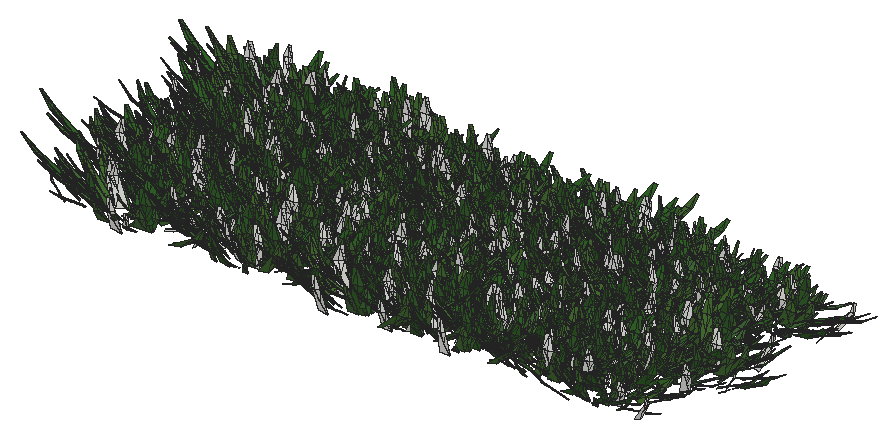
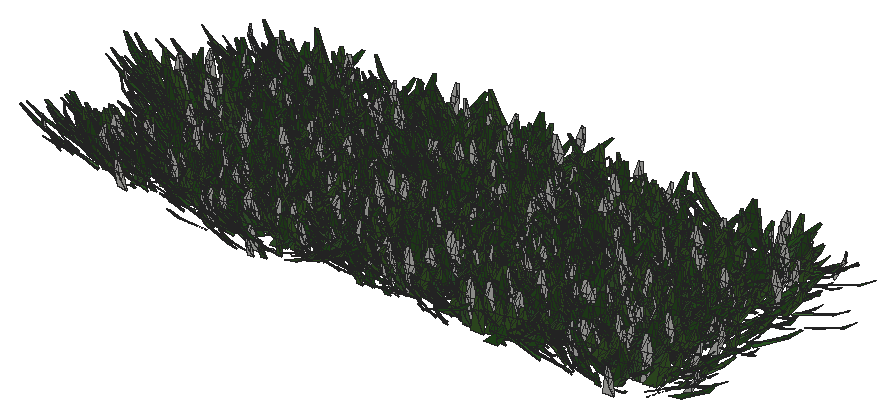
# SketchUp Ruby script. Lengths in inches.
U = 1.inch
M = Sketchup.active_model
def pt(a) = Geom::Point3d.new(a.map { |v| v * U })
def face(e, loops, mat)
  f = e.add_face(loops[0].map { |a| pt(a) })
  loops[1..].each { |l| e.add_face(l.map { |a| pt(a) }).erase! }
  f.material = f.back_material = mat if mat
  f
end
# faces: each face lists its corners as indices into pts; further lists are holes
def faces(e, pts, list, mat = nil) = list.each { |f| face(e, (f[0].is_a?(Array) ? f : [f]).map { |l| l.map { |i| pts[i] } }, mat) }
# xy, xz, yz: faces in a plane at the given z, y or x. An outline is a flat list of corners, or four numbers for a rectangle; further outlines are holes
def ring(l) = l.size == 4 ? [[l[0], l[1]], [l[2], l[1]], [l[2], l[3]], [l[0], l[3]]] : l.each_slice(2).to_a
def flat(e, list, mat, &to3) = list.each { |f| face(e, (f[0].is_a?(Array) ? f : [f]).map { |l| ring(l).map { |u, v| to3.(u, v) } }, mat) }
def xy(e, z, list, mat = nil) = flat(e, list, mat) { |x, y| [x, y, z] }
def xz(e, y, list, mat = nil) = flat(e, list, mat) { |x, z| [x, y, z] }
def yz(e, x, list, mat = nil) = flat(e, list, mat) { |y, z| [x, y, z] }
def lines(e, pts, list) = list.each { |a, b| e.add_line(pt(pts[a]), pt(pts[b])) }
# prism: a flat outline (further loops are holes) pulled along v
def prism(e, loops, v, mat = nil)
  f = face(e, loops, mat); d = Geom::Vector3d.new(v.map { |x| x * U })
  f.pushpull(f.normal.samedirection?(d) ? d.length : -d.length)
end
def box(e, o, s, mat = nil) = prism(e, [[o, [o[0] + s[0], o[1], o[2]], [o[0] + s[0], o[1] + s[1], o[2]], [o[0], o[1] + s[1], o[2]]]], [0, 0, s[2]], mat)
def at(x, y, z, deg = 0) = Geom::Transformation.translation(pt([x, y, z])) * Geom::Transformation.rotation(ORIGIN, Z_AXIS, deg.degrees)
def axes(o, x, y, z) = Geom::Transformation.new([*x, 0, *y, 0, *z, 0, *pt(o).to_a, 1])
def part(name) = M.definitions.add(name)
# library, detail: a bought-in or finely detailed component or shape, given as its bounding box
def library(name, o, s) = part(name).tap { |d| box(d.entities, o, s) }
def detail(e, o, s) = box(e.add_group.entities, o, s)
def put(e, d, t, mat = nil) = e.add_instance(d, t).tap { |i| i.material = mat if mat }
def group(e, t, mat = nil) = e.add_group.tap { |g| g.transformation = t; g.material = mat if mat }.entities
root = M.entities
M.materials.add("Material82").color = [68, 110, 58]
M.materials.add("Material83").color = [48, 90, 38]
M.materials.add("Material84").color = [68, 110, 48]
M.materials.add("Material85").color = [48, 90, 48]
M.materials.add("Material86").color = [58, 110, 58]
M.materials.add("Material87").color = [58, 90, 38]
M.materials.add("Material88").color = [68, 100, 58]
M.materials.add("Material89").color = [48, 100, 38]
c1 = part("grass00")
p = [[-0.6875,0.15,0],[-0.56,0.08,5.52],[-0.04,0.03,2.76],[0.48,-0.02,0],[0.35,-0.02,5.52],[-0.1,-0.14,5.52],
  [-0.12,0.65,8.37],[-0.42,0.65,8.37]]
faces(c1.entities,p,[[0,1,2,3],[3,2,4],[1,5,2],[5,4,2],[1,6,5],[4,5,6],[7,6,1]])
c2 = part("Group16\#1")
put(c2.entities,c1,axes([1.44,-0.61,-0.01],[0.05352,0.12609,0],[-0.10704,0.04543,0.07239],[0.06664,-0.02828,0.11628]),"Material85")
put(c2.entities,c1,axes([0.76,-0.15,-0.01],[0.04676,0.24062,0],[-0.23162,0.04501,0.06642],[0.0652,-0.01267,0.23595]),"Material82")
put(c2.entities,c1,axes([0.79,0.01,-0.01],[-0.00606,0.34651,0],[-0.34381,-0.00602,0.0432],[0.04319,0.00076,0.34386]))
put(c2.entities,c1,axes([1,0.23,-0.01],[-0.07192,0.31144,0],[-0.28722,-0.06632,0.1236],[0.12043,0.02781,0.29478]),"Material84")
put(c2.entities,c1,axes([1.66,0.77,-0.01],[-0.13828,0.29651,0],[-0.21551,-0.1005,0.22471],[0.20365,0.09498,0.23779]),"Material89")
put(c2.entities,c1,axes([0.6875,0.52,-0.01],[-0.18126,0.24051,0],[-0.22746,-0.17142,0.09788],[0.07817,0.05891,0.28481]),"Material84")
put(c2.entities,c1,axes([0.68,0.78,-0.01],[-0.215,0.18688,0],[-0.12385,-0.14248,0.21334],[0.13995,0.16101,0.18878]),"Material82")
put(c2.entities,c1,axes([0.56,1,-0.01],[-0.13756,0.07624,0],[-0.06159,-0.11112,0.0927],[0.04494,0.08108,0.12705]),"Material84")
put(c2.entities,c1,axes([0.2,0.64,-0.01],[-0.23729,0.07254,0],[-0.05711,-0.18681,0.153],[0.04473,0.14632,0.19535]),"Material89")
put(c2.entities,c1,axes([0.0625,0.72,-0.01],[-0.28874,0.02525,0],[-0.02179,-0.24916,0.14647],[0.01276,0.14591,0.25012]),"Material82")
put(c2.entities,c1,axes([-0.08,0.62,-0.01],[-0.34089,-0.04187,0],[0.03255,-0.26504,0.216],[-0.02633,0.21439,0.26703]),"Material89")
put(c2.entities,c1,axes([-0.34,0.98,-0.01],[-0.14314,-0.0493,0],[0.04397,-0.12769,0.06843],[-0.02228,0.0647,0.13505]),"Material89")
put(c2.entities,c1,axes([-0.87,1.45,-0.01],[-0.23488,-0.14114,0],[0.13761,-0.22901,0.06087],[-0.03135,0.05217,0.26717]))
put(c2.entities,c1,axes([-0.72,0.77,-0.01],[-0.14208,-0.13251,0],[0.07209,-0.0773,0.16301],[-0.11118,0.11922,0.1057]),"Material89")
put(c2.entities,c1,axes([-0.62,0.43,-0.01],[-0.14845,-0.21203,0],[0.18654,-0.13061,0.12304],[-0.10079,0.07057,0.22772]),"Material82")
put(c2.entities,c1,axes([-0.68,0.29,-0.01],[-0.13639,-0.32136,0],[0.31723,-0.13464,0.05579],[-0.05136,0.0218,0.34462]),"Material83")
put(c2.entities,c1,axes([-0.64,0.125,-0.01],[-0.0458,-0.23569,0],[0.22124,-0.043,0.08276],[-0.08124,0.01579,0.22538]),"Material86")
put(c2.entities,c1,axes([-1.6,-0.03,-0.01],[0.00576,-0.32897,0],[0.27526,0.00482,0.18018],[-0.18015,-0.00315,0.2753]),"Material84")
put(c2.entities,c1,axes([-1.36,-0.31,-0.01],[0.05718,-0.24765,0],[0.18172,0.04196,0.17267],[-0.16825,-0.03885,0.1865]),"Material89")
put(c2.entities,c1,axes([-1.54,-0.72,-0.01],[0.06537,-0.14017,0],[0.13555,0.06321,0.03939],[-0.0357,-0.01665,0.14956]))
put(c2.entities,c1,axes([-1.19,-0.9,-0.01],[0.09597,-0.12735,0],[0.11214,0.08451,0.07557],[-0.06035,-0.04548,0.14042]),"Material88")
put(c2.entities,c1,axes([-0.47,-0.54,-0.01],[0.11588,-0.10072,0],[0.0618,0.0711,0.12124],[-0.07953,-0.0915,0.0942]))
put(c2.entities,c1,axes([-0.47,-0.84,-0.01],[0.11927,-0.0661,0],[0.06603,0.11913,0.00646],[-0.00313,-0.00565,0.13621]),"Material84")
put(c2.entities,c1,axes([-0.38,-1.24,-0.01],[0.28037,-0.08571,0],[0.0618,0.20215,0.20315],[-0.05939,-0.19428,0.21139]),"Material88")
put(c2.entities,c1,axes([-0.06,-0.66,-0.01],[0.22719,-0.01987,0],[0.01247,0.14255,0.17758],[-0.01547,-0.17691,0.1431]),"Material87")
put(c2.entities,c1,axes([0.11,-0.89,-0.01],[0.14882,0.01828,0],[-0.01058,0.08611,0.12229],[0.01491,-0.12138,0.08676]),"Material85")
put(c2.entities,c1,axes([0.25,-0.72,-0.01],[0.20481,0.07053,0],[-0.06206,0.18022,0.10291],[0.03351,-0.0973,0.1906]),"Material85")
put(c2.entities,c1,axes([0.85,-1.42,-0.01],[0.16481,0.09904,0],[-0.09472,0.15762,0.05616],[0.02893,-0.04814,0.18389]),"Material84")
put(c2.entities,c1,axes([1.01,-1.09,-0.01],[0.21858,0.20385,0],[-0.17495,0.1876,0.15339],[0.10462,-0.11218,0.25652]),"Material89")
put(c2.entities,c1,axes([1.01,-0.71,-0.01],[0.08733,0.12473,0],[-0.06445,0.04512,0.13037],[0.1068,-0.07477,0.07867]),"Material85")
c3 = part("Group15\#1")
put(c3.entities,c2,at(0,0,0))
c4 = part("3darcstudiotree_grass00\#1")
put(c4.entities,c3,at(0,0,0))
put(root,c4,axes([1754.14,355.86,-34.17],[-3.58056,-0.39826,0],[0.95821,-1.33984,-0.015],[0.02011,-0.02812,1.30652]))
put(root,c4,axes([1754,346.47,-34.17],[-3.11874,1.35551,0],[-2.91461,-1.04296,-0.0082],[-0.03562,-0.01275,1.73071]))
put(root,c4,axes([1755.32,353.64,-34.17],[-3.23633,-0.50825,0],[1.72306,-1.70642,-0.01803],[0.03469,-0.03435,1.81493]))
put(root,c4,axes([1754.23,365.84,-34.17],[-1.77081,1.15286,0],[-3.98211,-0.9513,-0.05645],[-0.27396,-0.06545,1.97994]))
put(root,c4,axes([1754.09,364.16,-34.17],[2.97915,0.86965,0],[-2.38175,1.26898,-0.05487],[-0.15774,0.08404,1.44987]))
put(root,c4,axes([1755.32,361.99,-34.17],[3.36447,-1.00796,0],[2.1967,1.14039,-0.03309],[0.10605,0.05506,1.44206]))
put(root,c4,axes([1756.76,350.61,-34.17],[-3.57677,-1.09741,0],[2.84767,-1.44352,-0.06227],[0.15089,-0.07649,1.37168]))
put(root,c4,axes([1755.63,340.29,-34.17],[-0.9025,1.72738,0],[-3.54084,-0.28772,-0.03296],[-0.16809,-0.01366,1.411]))
put(root,c4,axes([1755.79,359.44,-34.17],[-1.59741,1.49736,0],[-3.22806,-0.5356,-0.02216],[-0.12937,-0.02146,1.66252]))
put(root,c4,axes([1756.57,348.21,-34.17],[-0.7508,1.54691,0],[-4.43091,-0.33447,-0.01652],[-0.07223,-0.00545,1.50529]))
put(root,c4,axes([1756.76,368.2,-34.17],[4.00478,-0.12141,0],[0.32544,1.66956,-0.03486],[0.01415,0.07259,1.68524]))
put(root,c4,axes([1757.17,357.11,-34.17],[3.83024,1.03121,0],[-2.22146,1.2833,-0.02215],[-0.08012,0.04629,1.8946]))
put(root,c4,axes([1760.06,353.15,-34.17],[-3.68156,-0.36216,0],[0.87025,-1.37591,-0.04204],[0.06138,-0.09705,1.62585]))
put(root,c4,axes([1759.72,339.76,-34.17],[-3.79448,1.12109,0],[-2.55555,-1.34526,-0.03017],[-0.0978,-0.05148,1.72726]))
put(root,c4,axes([1760.08,363.96,-34.17],[-3.10715,1.0196,0],[-2.89034,-1.36991,-0.01948],[-0.06651,-0.03152,1.80807]))
put(root,c4,axes([1760.29,361.45,-34.17],[3.31286,-0.55128,0],[1.80617,1.68812,-0.0407],[0.06877,0.06427,1.51351]))
put(root,c4,axes([1759.56,342.87,-34.17],[3.22227,0.82324,0],[-2.17222,1.32236,-0.01048],[-0.0296,0.01802,1.55517]))
put(root,c4,axes([1761.71,359.76,-34.17],[-4.269,-0.81813,0],[1.88917,-1.53314,-0.01545],[0.03796,-0.03081,1.8215]))
put(root,c4,axes([1760.42,355.12,-34.17],[0.15057,1.31453,0],[-3.70176,0.06595,-0.0329],[-0.23461,0.00418,1.98251]))
put(root,c4,axes([1760.38,347.21,-34.17],[-0.68682,1.71759,0],[-4.33467,-0.26958,-0.03641],[-0.15889,-0.00988,1.45326]))
put(root,c4,axes([1760.8,348.04,-34.17],[-1.33529,1.77622,0],[-3.16975,-0.37061,-0.00114],[-0.00828,-0.00097,1.86907]))
put(root,c4,axes([1760.34,356.7,-34.17],[1.34239,1.63135,0],[-4.02681,0.51535,-0.01715],[-0.07258,0.00929,1.41194]))
put(root,c4,axes([1761.43,366.09,-34.17],[-1.89402,1.2029,0],[-3.60721,-0.88336,-0.02009],[-0.09037,-0.02213,1.68525]))
put(root,c4,axes([1762.37,350.73,-34.17],[2.81192,0.87479,0],[-2.84329,1.42145,-0.06164],[-0.14998,0.07498,1.3518]))
put(root,c4,axes([1762.7,344.07,-34.17],[0.48103,1.53156,0],[-4.51259,0.22043,-0.03401],[-0.13914,0.0068,1.40523]))
put(root,c4,axes([1765.1875,360.96,-34.17],[-3.65599,0.07986,0],[-0.21877,-1.55768,-0.04105],[-0.01403,-0.0999,1.83253]))
put(root,c4,axes([1765.81,350.74,-34.17],[-2.36391,-1.30666,0],[2.88424,-0.81154,-0.04134],[0.24623,-0.06928,1.943]))
put(root,c4,axes([1765.08,345.07,-34.17],[-2.91503,0.96344,0],[-2.99535,-1.40954,-0.01682],[-0.05566,-0.02619,1.80026]))
put(root,c4,axes([1765.88,349.41,-34.17],[2.5477,-1.31265,0],[2.99582,0.90433,-0.00025],[0.00104,0.00031,1.45509]))
put(root,c4,axes([1765.71,363.8125,-34.17],[2.84002,-1.42543,0],[3.17904,0.98511,-0.04001],[0.1906,0.05906,1.83572]))
put(root,c4,axes([1765.02,357.56,-34.17],[4.10776,0.45174,0],[-0.96091,1.35899,-0.03867],[-0.06802,0.0962,1.75619]))
put(root,c4,axes([1766.99,355.55,-34.17],[-3.02492,-1.16677,0],[2.80082,-1.12934,-0.0483],[0.17838,-0.07192,1.58573]))
put(root,c4,axes([1767.42,342.88,-34.17],[1.67083,-1.60234,0],[3.7829,0.6135,-0.00107],[0.00454,0.00074,1.41133]))
put(root,c4,axes([1767.01,352.8125,-34.17],[-1.6341,1.38385,0],[-3.29524,-0.60518,-0.01596],[-0.09907,-0.01819,1.86544]))
put(root,c4,axes([1767.25,358.875,-34.17],[-1.88391,1.25543,0],[-3.77395,-0.8808,-0.04665],[-0.1806,-0.04215,1.47851]))
put(root,c4,axes([1767.61,346.4375,-34.17],[2.32026,0.93484,0],[-2.86948,1.10768,-0.01876],[-0.07886,0.03044,1.77063]))
put(root,c4,axes([1768.34,365.39,-34.17],[0.18236,1.53314,0],[-4.12116,0.07624,-0.04808],[-0.2649,0.0049,1.70557]))
put(root,c4,axes([1770.02,352.5,-34.17],[-3.65717,1.04753,0],[-2.10189,-1.14131,-0.02785],[-0.11272,-0.06121,1.84622]))
put(root,c4,axes([1770,363.99,-34.17],[2.69686,-1.18339,0],[2.47302,0.87653,-0.01288],[0.05957,0.02111,1.54961]))
put(root,c4,axes([1770.875,357.19,-34.17],[-3.84397,-0.38485,0],[1.07963,-1.67717,-0.00944],[0.01366,-0.02122,1.93444]))
put(root,c4,axes([1770.72,350.7,-34.17],[-1.0379,-1.53247,0],[3.79206,-0.39944,-0.04991],[0.21721,-0.02288,1.32514]))
put(root,c4,axes([1770.86,348.89,-34.17],[1.97874,-1.59829,0],[3.60248,0.69366,-0.03421],[0.19371,0.0373,1.89316]))
put(root,c4,axes([1770.07,366.47,-34.17],[1.07752,1.49554,0],[-4.17421,0.46775,-0.01918],[-0.10688,0.01198,1.88463]))
put(root,c4,axes([1772.22,346.51,-34.17],[-0.05891,-1.32731,0],[4.1482,-0.02863,-0.04239],[0.194,-0.00134,1.42343]))
put(root,c4,axes([1773.02,362.16,-34.17],[-0.12973,-1.5282,0],[4.23676,-0.05594,-0.02714],[0.12341,-0.00163,1.44559]))
put(root,c4,axes([1772.64,340.54,-34.17],[2.6038,-1.3441,0],[3.00735,0.90609,-0.00592],[0.02965,0.00893,1.78738]))
put(root,c4,axes([1773.5,341.58,-34.17],[-2.61082,-1.14432,0],[2.90627,-1.03127,-0.02928],[0.10098,-0.03583,1.35967]))
put(root,c4,axes([1772.72,367.58,-34.17],[-0.14307,1.431,0],[-4.32963,-0.06732,-0.01193],[-0.07261,-0.00113,1.97773]))
put(root,c4,axes([1773.49,355.81,-34.17],[-0.09674,1.30199,0],[-3.40883,-0.03939,-0.04664],[-0.25839,-0.00299,1.41669]))
put(root,c4,axes([1773.43,360.35,-34.17],[2.79143,1.2628,0],[-2.51561,0.86486,-0.0286],[-0.15611,0.05367,1.81122]))
put(root,c4,axes([1773.68,344.74,-34.17],[-0.55757,1.6642,0],[-4.56304,-0.23777,-0.03274],[-0.13576,-0.00707,1.44297]))
put(root,c4,axes([1775.76,359.68,-34.17],[-3.21861,0.39731,0],[-1.33805,-1.68585,-0.0251],[-0.03563,-0.04489,1.59541]))
put(root,c4,axes([1775.82,345.94,-34.17],[0.77539,1.49335,0],[-4.15697,0.3357,-0.02758],[-0.13791,0.01114,1.62317]))
put(root,c4,axes([1776.09,361.16,-34.17],[0.83918,1.59477,0],[-3.76377,0.30803,-0.00381],[-0.02098,0.00172,1.62105]))
put(root,c4,axes([1777.85,354.72,-34.17],[-4.69627,0.21945,0],[-0.46002,-1.53114,-0.03012],[-0.01578,-0.05252,1.30483]))
put(root,c4,axes([1776.76,341.91,-34.17],[-1.57534,1.27293,0],[-3.92925,-0.75629,-0.02753],[-0.13899,-0.02675,1.84121]))
put(root,c4,axes([1777.14,344.88,-34.17],[2.05797,-1.09603,0],[2.87826,0.84054,-0.04843],[0.25021,0.07307,1.72564]))
put(root,c4,axes([1778.17,364.21,-34.17],[1.23956,-1.20185,0],[3.42028,0.54865,-0.0011],[0.00669,0.00107,1.80895]))
put(root,c4,axes([1778.22,352.85,-34.17],[0.89327,-1.81074,0],[4.0321,0.30937,-0.02432],[0.12035,0.00923,1.55217]))
put(root,c4,axes([1779.1,350.68,-34.17],[0.20119,-1.37174,0],[3.84475,0.0877,-0.03098],[0.16829,0.00384,1.57088]))
put(root,c4,axes([1779.46,349.46,-34.17],[-0.37192,-1.4591,0],[3.79295,-0.15037,-0.02999],[0.19954,-0.00791,1.91089]))
put(root,c4,axes([1779.18,365.71,-34.17],[2.01038,-1.40201,0],[3.67214,0.81896,-0.04614],[0.18867,0.04208,1.48544]))
put(root,c4,axes([1779.42,356.7,-34.17],[4.6177,0.37892,0],[-0.96466,1.82835,-0.01168],[-0.00936,0.01774,1.39591]))
put(root,c4,axes([1782.6,362.125,-34.17],[-2.89327,-0.98526,0],[2.3422,-1.06973,-0.01919],[0.0931,-0.04252,1.99409]))
put(root,c4,axes([1782.85,347.22,-34.17],[-3.01308,-1.39849,0],[3.33443,-1.11734,-0.06095],[0.24941,-0.08358,1.76096]))
put(root,c4,axes([1782.6875,351.39,-34.17],[1.17396,-1.50467,0],[4.45897,0.54108,-0.02541],[0.10297,0.01249,1.48254]))
put(root,c4,axes([1783.38,357.33,-34.17],[-3.89542,-0.50736,0],[1.22292,-1.46031,-0.04962],[0.09609,-0.11475,1.8049]))
put(root,c4,axes([1782.76,349.24,-34.17],[-2.84312,0.65512,0],[-2.18872,-1.47733,-0.05376],[-0.11522,-0.07777,1.38154]))
put(root,c4,axes([1782.27,360.03,-34.17],[-0.91872,1.71096,0],[-4.38194,-0.36595,-0.05285],[-0.26515,-0.02214,1.72177]))
put(root,c4,axes([1783,342.36,-34.17],[4.14821,-0.06928,0],[0.17152,1.59736,-0.02002],[0.00473,0.044,1.69539]))
put(root,c4,axes([1784.86,354.59,-34.17],[-3.82686,-0.23596,0],[0.71117,-1.79387,-0.04342],[0.03245,-0.08186,1.66984]))
put(root,c4,axes([1783.78,365.83,-34.17],[-1.95951,1.68141,0],[-3.84767,-0.6974,-0.02861],[-0.15441,-0.02799,1.88512]))
put(root,c4,axes([1784.91,352.36,-34.17],[-3.45153,-0.0864,0],[0.28769,-1.78743,-0.04372],[0.01068,-0.06634,1.31241]))
put(root,c4,axes([1784.3,363.9,-34.17],[1.28845,1.74913,0],[-3.19455,0.36599,-0.00931],[-0.04886,0.0056,1.3628]))
put(root,c4,axes([1785.07,345.01,-34.17],[3.2366,-0.57131,0],[1.58048,1.39258,-0.04939],[0.12568,0.11074,1.80606]))
put(root,c4,axes([1787.17,366.41,-34.17],[-3.18632,0.63668,0],[-1.6075,-1.25121,-0.00642],[-0.0144,-0.01121,1.3229]))
put(root,c4,axes([1787.8,341.95,-34.17],[-3.56938,-0.43544,0],[1.36231,-1.73682,-0.06046],[0.07694,-0.09809,1.48798]))
put(root,c4,axes([1787.34,339.75,-34.17],[-3.08205,1.07293,0],[-3.11637,-1.39229,-0.01862],[-0.0666,-0.02976,1.90809]))
put(root,c4,axes([1787.31,357.74,-34.17],[-2.17882,1.11223,0],[-3.27984,-0.99929,-0.01374],[-0.05934,-0.01808,1.69563]))
put(root,c4,axes([1786.97,346.79,-34.17],[-1.12838,1.66356,0],[-4.06225,-0.42855,-0.00132],[-0.00752,-0.00079,1.858]))
put(root,c4,axes([1786.58,364.08,-34.17],[3.24771,1.22669,0],[-3.17033,1.30544,-0.01961],[-0.06543,0.02694,1.65716]))
put(root,c4,axes([1788.43,344.16,-34.17],[-3.65901,0.17551,0],[-0.56536,-1.83311,-0.00408],[-0.00246,-0.00797,1.74968]))
put(root,c4,axes([1788.16,361.08,-34.17],[2.96136,1.19987,0],[-3.11013,1.19384,-0.004],[-0.01667,0.0064,1.89371]))
put(root,c4,axes([1789.96,351.35,-34.17],[-4.14748,0.25836,0],[-0.59761,-1.49206,-0.01239],[-0.00958,-0.02393,1.42361]))
put(root,c4,axes([1788.7,348.75,-34.17],[4.21182,0.14848,0],[-0.32581,1.4374,-0.01038],[-0.00654,0.02884,1.94021]))
put(root,c4,axes([1788.84,353.38,-34.17],[1.10995,1.51966,0],[-3.58981,0.40779,-0.02733],[-0.15418,0.01751,1.64375]))
put(root,c4,axes([1790.02,360.39,-34.17],[4.19014,0.72772,0],[-1.46084,1.30821,-0.04159],[-0.08773,0.07856,1.42181]))
put(root,c4,axes([1792.06,348.02,-34.17],[-1.84068,-1.59832,0],[3.91902,-0.70195,-0.02239],[0.11993,-0.02148,1.89813]))
put(root,c4,axes([1790.59,354.66,-34.17],[0.99879,1.74855,0],[-3.87665,0.3444,-0.04632],[-0.24296,0.02158,1.6013]))
put(root,c4,axes([1793.68,341.84,-34.17],[-0.45548,-1.68091,0],[3.45741,-0.14571,-0.01446],[0.0889,-0.00375,1.61179]))
put(root,c4,axes([1793.13,340.49,-34.17],[-3.13157,0.80525,0],[-2.19448,-1.32731,-0.02083],[-0.06068,-0.0367,1.60618]))
put(root,c4,axes([1794.38,361.875,-34.17],[-3.37995,-1.26993,0],[3.24999,-1.34532,-0.03405],[0.09733,-0.04029,1.46358]))
put(root,c4,axes([1792.41,353.72,-34.17],[1.40547,1.51439,0],[-4.0139,0.57938,-0.03042],[-0.14333,0.02069,1.60735]))
put(root,c4,axes([1794.02,346.53,-34.17],[-0.09951,1.54184,0],[-3.8951,-0.0391,-0.03168],[-0.18001,-0.00181,1.66016]))
put(root,c4,axes([1794.5625,364.19,-34.17],[3.13004,-0.71111,0],[2.12935,1.45771,-0.00508],[0.01244,0.00852,1.56982]))
put(root,c4,axes([1794.125,359.87,-34.17],[1.71903,1.73474,0],[-3.69921,0.57012,-0.05423],[-0.23247,0.03583,1.37014]))
put(root,c4,axes([1795.55,355.33,-34.17],[1.52517,-1.72025,0],[3.68343,0.50792,-0.01723],[0.07984,0.01101,1.43549]))
put(root,c4,axes([1795.1,344.76,-34.17],[-2.42659,1.57566,0],[-3.75552,-0.89953,-0.06137],[-0.23264,-0.05572,1.46064]))
put(root,c4,axes([1794.79,350.39,-34.17],[3.59244,-0.46408,0],[1.16578,1.40355,-0.03684],[0.0661,0.07959,1.61813]))
put(root,c4,axes([1795.9375,356.9,-34.17],[-3.02925,1.34013,0],[-2.7234,-0.95744,-0.02096],[-0.09613,-0.0338,1.6805]))
put(root,c4,axes([1795.79,365.84,-34.17],[2.66376,1.48543,0],[-3.56736,0.99495,-0.03132],[-0.13982,0.039,1.7905]))
put(root,c4,axes([1798.8,367.96,-34.17],[-1.65449,-1.67632,0],[3.5536,-0.54549,-0.00938],[0.04968,-0.00763,1.62403]))
put(root,c4,axes([1798.91,357.72,-34.17],[-2.10435,-1.3155,0],[3.64518,-0.9069,-0.04882],[0.17684,-0.044,1.38366]))
put(root,c4,axes([1798.07,352.34,-34.17],[3.93831,-0.79818,0],[2.14355,1.64496,-0.04443],[0.08068,0.06192,1.39643]))
put(root,c4,axes([1799.32,361.03,-34.17],[-2.03778,-1.0951,0],[3.7049,-1.07224,-0.05528],[0.23064,-0.06675,1.78248]))
put(root,c4,axes([1799.34,360.06,-34.17],[-3.67688,-0.6634,0],[1.45076,-1.25058,-0.02741],[0.08145,-0.07021,1.86713]))
put(root,c4,axes([1797.71,364.18,-34.17],[3.8654,0.35733,0],[-0.81256,1.36706,-0.007],[-0.00937,0.01576,1.56436]))
put(root,c4,axes([1799.72,348.66,-34.17],[-3.021,-0.6477,0],[1.60996,-1.16789,-0.02167],[0.0547,-0.03968,1.33527]))
put(root,c4,axes([1799.32,340.22,-34.17],[-3.52536,0.66718,0],[-1.57507,-1.29441,-0.02803],[-0.08559,-0.07034,1.92571]))
put(root,c4,axes([1798.89,355.35,-34.17],[3.86172,-0.56351,0],[1.21864,1.29888,-0.04569],[0.10723,0.11428,1.78027]))
put(root,c4,axes([1799.68,350.49,-34.17],[2.47969,-0.8558,0],[2.79846,1.26111,-0.0129],[0.03707,0.01671,1.39029]))
put(root,c4,axes([1799.4,366.86,-34.17],[3.77184,-0.74152,0],[2.04611,1.61872,-0.00236],[0.0043,0.00341,1.40454]))
put(root,c4,axes([1799.35,344,-34.17],[4.4523,-0.10128,0],[0.21715,1.4846,-0.03809],[0.01394,0.09529,1.79573]))
put(root,c4,axes([1799.78,342.59,-34.17],[3.96943,-0.89247,0],[1.86138,1.2876,-0.05304],[0.17378,0.12021,1.86337]))
put(root,c4,axes([1801.2,346.2,-34.17],[-0.06079,-1.40056,0],[3.30003,-0.02228,-0.01279],[0.0855,-0.00058,1.65408]))
put(root,c4,axes([1803.14,347.09,-34.17],[-0.30634,-1.35211,0],[4.22133,-0.14875,-0.01785],[0.10663,-0.00376,1.90542]))
put(root,c4,axes([1803.23,347.87,-34.17],[0.00917,-1.7323,0],[3.83355,0.00316,-0.00952],[0.04811,0.00004,1.45276]))
put(root,c4,axes([1803.17,363.77,-34.17],[3.51422,-0.54071,0],[1.19989,1.21289,-0.03886],[0.08676,0.0877,1.52001]))
put(root,c4,axes([1803.97,343.89,-34.17],[0.66388,1.42145,0],[-3.998,0.29041,-0.0472],[-0.22325,0.01622,1.46547]))
put(root,c4,axes([1804.07,366.42,-34.17],[2.60904,1.49403,0],[-2.88542,0.78369,-0.04649],[-0.18984,0.05156,1.30192]))
put(root,c4,axes([1804.18,354.63,-34.17],[3.83063,0.28141,0],[-0.63066,1.33518,-0.03922],[-0.04064,0.08605,1.46066]))
put(root,c4,axes([1806.72,359.01,-34.17],[-2.44222,-1.21448,0],[3.27109,-1.02306,-0.01126],[0.03735,-0.01168,1.32461]))
put(root,c4,axes([1806.39,353.71,-34.17],[-3.39135,-0.3159,0],[0.83318,-1.39116,-0.01801],[0.02035,-0.03397,1.33554]))
put(root,c4,axes([1806.27,350.4375,-34.17],[-1.25644,-1.35671,0],[3.16457,-0.45581,-0.03784],[0.23357,-0.03364,1.65933]))
put(root,c4,axes([1806.82,361.55,-34.17],[-4.6912,-0.24024,0],[0.57575,-1.74859,-0.02421],[0.01544,-0.0469,1.66024]))
put(root,c4,axes([1805.93,341.97,-34.17],[3.97766,0.18345,0],[-0.40911,1.37962,-0.0104],[-0.00856,0.02886,1.87036]))
put(root,c4,axes([1806.875,357.85,-34.17],[3.80429,-0.95187,0],[2.21902,1.37934,-0.04672],[0.14892,0.09257,1.84728]))
put(root,c4,axes([1809.23,361.2,-34.17],[2.08515,-1.11593,0],[3.14779,0.91479,-0.04551],[0.20545,0.05971,1.64335]))
put(root,c4,axes([1809.26,355.11,-34.17],[-2.84594,1.17329,0],[-3.06349,-1.15571,-0.01205],[-0.05136,-0.01938,1.87482]))
put(root,c4,axes([1810.3,345.09,-34.17],[-4.1718,-0.04402,0],[0.1133,-1.66995,-0.01377],[0.00192,-0.02825,1.65227]))
put(root,c4,axes([1810.8125,350.47,-34.17],[-3.23677,-0.61439,0],[2.0349,-1.66734,-0.00367],[0.00726,-0.00595,1.60507]))
put(root,c4,axes([1810.42,341.94,-34.17],[0.66157,-1.84804,0],[3.88634,0.21638,-0.01886],[0.11067,0.00616,1.74385]))
put(root,c4,axes([1809.4375,365.62,-34.17],[3.70848,0.20038,0],[-0.48617,1.3994,-0.00884],[-0.00845,0.02433,1.89082]))
put(root,c4,axes([1810.94,348.4375,-34.17],[3.82795,-0.89848,0],[2.12017,1.40489,-0.02674],[0.0662,0.04387,1.50406]))
put(root,c4,axes([1811.9,363.38,-34.17],[-3.70161,0.1835,0],[-0.55617,-1.74492,-0.04842],[-0.0352,-0.11043,1.94818]))
put(root,c4,axes([1811.09,360.07,-34.17],[4.60425,0.18746,0],[-0.4763,1.81947,-0.06196],[-0.02818,0.10763,1.53928]))
put(root,c4,axes([1811.3125,346.01,-34.17],[3.66376,0.25232,0],[-0.75626,1.7079,-0.04039],[-0.02947,0.06656,1.39779]))
put(root,c4,axes([1811.56,357.88,-34.17],[3.38223,0.96892,0],[-2.45655,1.33368,-0.05492],[-0.16887,0.09168,1.63919]))
put(root,c4,axes([1812.46,353.62,-34.17],[3.17823,1.19717,0],[-2.46254,1.01678,-0.00574],[-0.02103,0.00868,1.41814]))
put(root,c4,axes([1815.33,342.06,-34.17],[-4.20115,-0.27572,0],[0.6063,-1.43684,-0.03971],[0.03476,-0.08238,1.4765]))
put(root,c4,axes([1814.73,348.79,-34.17],[3.03154,-1.30842,0],[2.70015,0.973,-0.04297],[0.17128,0.06172,1.48019]))
put(root,c4,axes([1814.64,351.42,-34.17],[4.0708,-0.43574,0],[1.12817,1.63922,-0.0215],[0.0298,0.0433,1.70776]))
put(root,c4,axes([1814.96,362.3125,-34.17],[3.98961,-0.74286,0],[1.49364,1.24762,-0.01833],[0.03992,0.03334,1.33779]))
put(root,c4,axes([1814.89,364.36,-34.17],[-1.90909,1.29111,0],[-3.77719,-0.86865,-0.00159],[-0.00678,-0.00156,1.61385]))
put(root,c4,axes([1816.95,340.62,-34.17],[-2.56515,-0.8375,0],[2.7288,-1.2999,-0.02106],[0.06081,-0.02897,1.45262]))
put(root,c4,axes([1814.93,358.84,-34.17],[1.21271,1.28553,0],[-4.16441,0.61099,-0.01219],[-0.04469,0.00656,1.30286]))
put(root,c4,axes([1816.17,352.52,-34.17],[-3.04036,1.06501,0],[-2.34315,-1.04035,-0.02123],[-0.07304,-0.03243,1.37003]))
put(root,c4,axes([1816.39,358.19,-34.17],[1.27723,-1.67859,0],[3.60633,0.42678,-0.0465],[0.22987,0.0272,1.45674]))
put(root,c4,axes([1815.46,346.06,-34.17],[4.09443,-0.06366,0],[0.15428,1.54325,-0.03451],[0.00867,0.0867,1.8714]))
put(root,c4,axes([1815.4,344.07,-34.17],[3.43879,0.48398,0],[-1.47194,1.62658,-0.03925],[-0.05225,0.05774,1.29995]))
put(root,c4,axes([1817.81,354.84,-34.17],[-0.06785,-1.57512,0],[4.70678,-0.03153,-0.0635],[0.34719,-0.00233,1.92948]))
put(root,c4,axes([1818.26,365.89,-34.17],[3.5964,-0.66598,0],[1.43149,1.20228,-0.03796],[0.09777,0.08212,1.52986]))
put(root,c4,axes([1820.2,348.71,-34.17],[-3.83088,0.01586,0],[-0.04003,-1.50367,-0.01485],[-0.00089,-0.03334,1.62647]))
put(root,c4,axes([1820.71,362.45,-34.17],[-1.26463,-1.25515,0],[3.81596,-0.59798,-0.04918],[0.19961,-0.03128,1.34418]))
put(root,c4,axes([1821.15,364.37,-34.17],[0.54946,-1.30633,0],[4.42126,0.28923,-0.06063],[0.27406,0.01793,1.53907]))
put(root,c4,axes([1821.84,352.46,-34.17],[1.45773,-1.41559,0],[3.72691,0.5969,-0.04502],[0.25742,0.04123,1.86083]))
